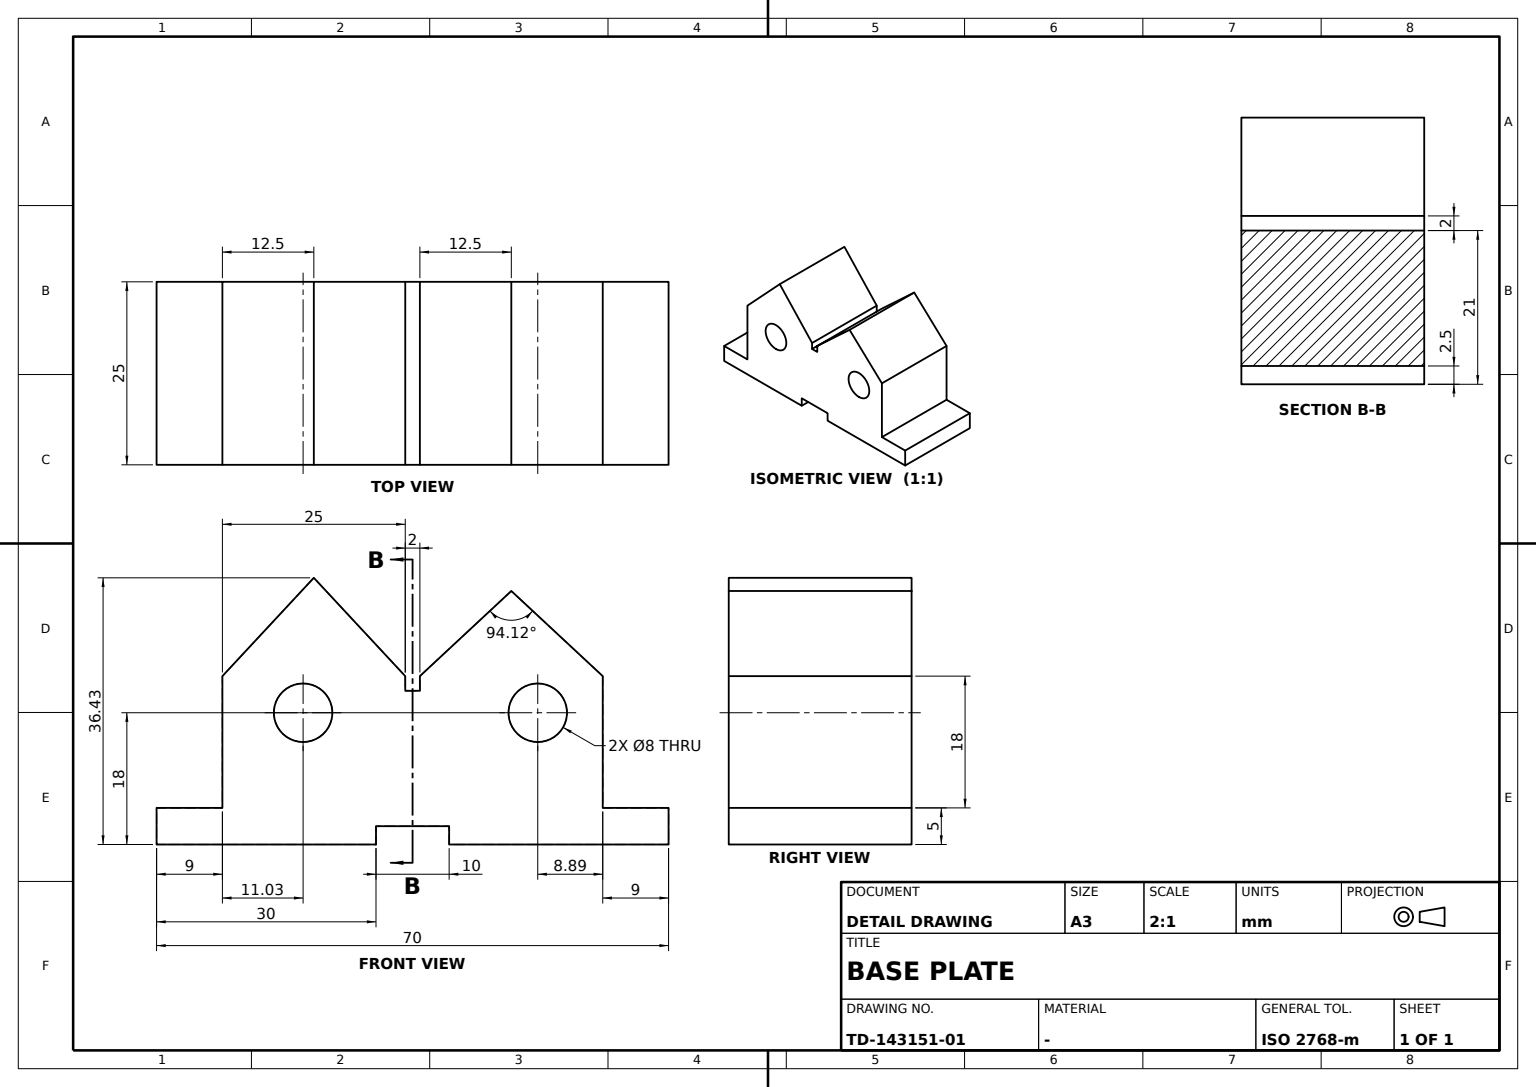
ISO-10303-21;
HEADER;
FILE_DESCRIPTION((''),'2;1');
FILE_NAME('','',(''),(''),'','','');
FILE_SCHEMA(('AUTOMOTIVE_DESIGN'));
ENDSEC;
DATA;
#1=APPLICATION_CONTEXT('');
#2=PRODUCT_CONTEXT('',#1,'mechanical');
#3=PRODUCT('','','',(#2));
#4=PRODUCT_DEFINITION_FORMATION('','',#3);
#5=PRODUCT_DEFINITION_CONTEXT('',#1,'design');
#6=PRODUCT_DEFINITION('','',#4,#5);
#7=PRODUCT_DEFINITION_SHAPE('','',#6);
#8=(LENGTH_UNIT()NAMED_UNIT(*)SI_UNIT(.MILLI.,.METRE.));
#9=(NAMED_UNIT(*)PLANE_ANGLE_UNIT()SI_UNIT($,.RADIAN.));
#10=(NAMED_UNIT(*)SI_UNIT($,.STERADIAN.)SOLID_ANGLE_UNIT());
#11=UNCERTAINTY_MEASURE_WITH_UNIT(LENGTH_MEASURE(0.005),#8,'distance_accuracy_value','');
#12=(GEOMETRIC_REPRESENTATION_CONTEXT(3)GLOBAL_UNCERTAINTY_ASSIGNED_CONTEXT((#11))GLOBAL_UNIT_ASSIGNED_CONTEXT((#8,#9,#10))REPRESENTATION_CONTEXT('',''));
#13=CARTESIAN_POINT('',(-25.,-14.966636,2.5));
#14=VERTEX_POINT('',#13);
#15=CARTESIAN_POINT('',(-25.,-14.966636,6.5));
#16=DIRECTION('',(1.,0.,0.));
#17=DIRECTION('',(0.,0.,-1.));
#18=AXIS2_PLACEMENT_3D('',#15,#16,#17);
#19=CIRCLE('',#18,4.);
#20=EDGE_CURVE('',#14,#14,#19,.T.);
#21=ORIENTED_EDGE('',*,*,#20,.F.);
#22=EDGE_LOOP('',(#21));
#23=FACE_BOUND('',#22,.T.);
#24=CARTESIAN_POINT('',(0.,-14.966636,2.5));
#25=VERTEX_POINT('',#24);
#26=CARTESIAN_POINT('',(0.,-14.966636,6.5));
#27=AXIS2_PLACEMENT_3D('',#26,#16,#17);
#28=CIRCLE('',#27,4.);
#29=EDGE_CURVE('',#25,#25,#28,.T.);
#30=ORIENTED_EDGE('',*,*,#29,.T.);
#31=EDGE_LOOP('',(#30));
#32=FACE_BOUND('',#31,.T.);
#33=CARTESIAN_POINT('',(-13.16,-14.966636,6.5));
#34=DIRECTION('',(0.,1.,0.));
#35=AXIS2_PLACEMENT_3D('',#33,#16,#34);
#36=CYLINDRICAL_SURFACE('',#35,4.);
#37=ADVANCED_FACE('',(#23,#32),#36,.F.);
#38=CARTESIAN_POINT('',(0.,35.,-11.5));
#39=VERTEX_POINT('',#38);
#40=CARTESIAN_POINT('',(0.,35.,-6.5));
#41=VERTEX_POINT('',#40);
#42=DIRECTION('',(0.,0.,1.));
#43=VECTOR('',#42,1000.);
#44=LINE('',#38,#43);
#45=EDGE_CURVE('',#39,#41,#44,.T.);
#46=ORIENTED_EDGE('',*,*,#45,.F.);
#47=CARTESIAN_POINT('',(-25.,35.,-11.5));
#48=VERTEX_POINT('',#47);
#49=DIRECTION('',(-1.,0.,0.));
#50=VECTOR('',#49,1000.);
#51=LINE('',#38,#50);
#52=EDGE_CURVE('',#39,#48,#51,.T.);
#53=ORIENTED_EDGE('',*,*,#52,.T.);
#54=CARTESIAN_POINT('',(-25.,35.,-6.5));
#55=VERTEX_POINT('',#54);
#56=LINE('',#47,#43);
#57=EDGE_CURVE('',#48,#55,#56,.T.);
#58=ORIENTED_EDGE('',*,*,#57,.T.);
#59=LINE('',#40,#50);
#60=EDGE_CURVE('',#41,#55,#59,.T.);
#61=ORIENTED_EDGE('',*,*,#60,.F.);
#62=EDGE_LOOP('',(#46,#53,#58,#61));
#63=FACE_BOUND('',#62,.T.);
#64=DIRECTION('',(0.,-1.,0.));
#65=AXIS2_PLACEMENT_3D('',#38,#64,#42);
#66=PLANE('',#65);
#67=ADVANCED_FACE('',(#63),#66,.F.);
#68=CARTESIAN_POINT('',(0.,26.,-6.5));
#69=VERTEX_POINT('',#68);
#70=VECTOR('',#64,1000.);
#71=LINE('',#40,#70);
#72=EDGE_CURVE('',#41,#69,#71,.T.);
#73=ORIENTED_EDGE('',*,*,#72,.F.);
#74=ORIENTED_EDGE('',*,*,#60,.T.);
#75=CARTESIAN_POINT('',(-25.,26.,-6.5));
#76=VERTEX_POINT('',#75);
#77=LINE('',#54,#70);
#78=EDGE_CURVE('',#55,#76,#77,.T.);
#79=ORIENTED_EDGE('',*,*,#78,.T.);
#80=LINE('',#68,#50);
#81=EDGE_CURVE('',#69,#76,#80,.T.);
#82=ORIENTED_EDGE('',*,*,#81,.F.);
#83=EDGE_LOOP('',(#73,#74,#79,#82));
#84=FACE_BOUND('',#83,.T.);
#85=AXIS2_PLACEMENT_3D('',#40,#17,#64);
#86=PLANE('',#85);
#87=ADVANCED_FACE('',(#84),#86,.F.);
#88=ORIENTED_EDGE('',*,*,#29,.F.);
#89=EDGE_LOOP('',(#88));
#90=FACE_BOUND('',#89,.T.);
#91=CARTESIAN_POINT('',(0.,-1.,11.5));
#92=VERTEX_POINT('',#91);
#93=CARTESIAN_POINT('',(0.,-1.,9.5));
#94=VERTEX_POINT('',#93);
#95=CARTESIAN_POINT('',(0.,-1.,0.));
#96=VECTOR('',#17,1000.);
#97=LINE('',#95,#96);
#98=EDGE_CURVE('',#92,#94,#97,.T.);
#99=ORIENTED_EDGE('',*,*,#98,.F.);
#100=CARTESIAN_POINT('',(0.,-13.5,24.931745));
#101=VERTEX_POINT('',#100);
#102=DIRECTION('',(0.,0.681260343,-0.732041218));
#103=VECTOR('',#102,1000.);
#104=LINE('',#100,#103);
#105=EDGE_CURVE('',#101,#92,#104,.T.);
#106=ORIENTED_EDGE('',*,*,#105,.F.);
#107=CARTESIAN_POINT('',(0.,-26.,11.5));
#108=VERTEX_POINT('',#107);
#109=DIRECTION('',(0.,0.681260343,0.732041218));
#110=VECTOR('',#109,1000.);
#111=LINE('',#107,#110);
#112=EDGE_CURVE('',#108,#101,#111,.T.);
#113=ORIENTED_EDGE('',*,*,#112,.F.);
#114=CARTESIAN_POINT('',(0.,-26.,-6.5));
#115=VERTEX_POINT('',#114);
#116=LINE('',#107,#96);
#117=EDGE_CURVE('',#108,#115,#116,.T.);
#118=ORIENTED_EDGE('',*,*,#117,.T.);
#119=CARTESIAN_POINT('',(0.,-35.,-6.5));
#120=VERTEX_POINT('',#119);
#121=EDGE_CURVE('',#115,#120,#71,.T.);
#122=ORIENTED_EDGE('',*,*,#121,.T.);
#123=CARTESIAN_POINT('',(0.,-35.,-11.5));
#124=VERTEX_POINT('',#123);
#125=LINE('',#119,#96);
#126=EDGE_CURVE('',#120,#124,#125,.T.);
#127=ORIENTED_EDGE('',*,*,#126,.T.);
#128=CARTESIAN_POINT('',(0.,-5.,-11.5));
#129=VERTEX_POINT('',#128);
#130=VECTOR('',#34,1000.);
#131=LINE('',#123,#130);
#132=EDGE_CURVE('',#124,#129,#131,.T.);
#133=ORIENTED_EDGE('',*,*,#132,.T.);
#134=CARTESIAN_POINT('',(0.,-5.,-9.));
#135=VERTEX_POINT('',#134);
#136=LINE('',#128,#43);
#137=EDGE_CURVE('',#129,#135,#136,.T.);
#138=ORIENTED_EDGE('',*,*,#137,.T.);
#139=CARTESIAN_POINT('',(0.,5.,-9.));
#140=VERTEX_POINT('',#139);
#141=LINE('',#134,#130);
#142=EDGE_CURVE('',#135,#140,#141,.T.);
#143=ORIENTED_EDGE('',*,*,#142,.T.);
#144=CARTESIAN_POINT('',(0.,5.,-11.5));
#145=VERTEX_POINT('',#144);
#146=LINE('',#144,#96);
#147=EDGE_CURVE('',#140,#145,#146,.T.);
#148=ORIENTED_EDGE('',*,*,#147,.T.);
#149=EDGE_CURVE('',#145,#39,#131,.T.);
#150=ORIENTED_EDGE('',*,*,#149,.T.);
#151=ORIENTED_EDGE('',*,*,#45,.T.);
#152=ORIENTED_EDGE('',*,*,#72,.T.);
#153=CARTESIAN_POINT('',(0.,26.,11.5));
#154=VERTEX_POINT('',#153);
#155=LINE('',#68,#43);
#156=EDGE_CURVE('',#69,#154,#155,.T.);
#157=ORIENTED_EDGE('',*,*,#156,.T.);
#158=CARTESIAN_POINT('',(0.,13.5,23.132889));
#159=VERTEX_POINT('',#158);
#160=DIRECTION('',(0.,0.732041218,-0.681260343));
#161=VECTOR('',#160,1000.);
#162=LINE('',#158,#161);
#163=EDGE_CURVE('',#159,#154,#162,.T.);
#164=ORIENTED_EDGE('',*,*,#163,.F.);
#165=CARTESIAN_POINT('',(0.,1.,11.5));
#166=VERTEX_POINT('',#165);
#167=DIRECTION('',(0.,0.732041218,0.681260343));
#168=VECTOR('',#167,1000.);
#169=LINE('',#165,#168);
#170=EDGE_CURVE('',#166,#159,#169,.T.);
#171=ORIENTED_EDGE('',*,*,#170,.F.);
#172=CARTESIAN_POINT('',(0.,1.,9.5));
#173=VERTEX_POINT('',#172);
#174=LINE('',#172,#43);
#175=EDGE_CURVE('',#173,#166,#174,.T.);
#176=ORIENTED_EDGE('',*,*,#175,.F.);
#177=LINE('',#93,#130);
#178=EDGE_CURVE('',#94,#173,#177,.T.);
#179=ORIENTED_EDGE('',*,*,#178,.F.);
#180=EDGE_LOOP('',(#99,#106,#113,#118,#122,#127,#133,#138,#143,#148,#150,#151,#152,#157,#164,#171,#176,#179));
#181=FACE_BOUND('',#180,.T.);
#182=CARTESIAN_POINT('',(0.,17.114063,2.5));
#183=VERTEX_POINT('',#182);
#184=CARTESIAN_POINT('',(0.,17.114063,6.5));
#185=AXIS2_PLACEMENT_3D('',#184,#16,#17);
#186=CIRCLE('',#185,4.);
#187=EDGE_CURVE('',#183,#183,#186,.T.);
#188=ORIENTED_EDGE('',*,*,#187,.F.);
#189=EDGE_LOOP('',(#188));
#190=FACE_BOUND('',#189,.T.);
#191=CARTESIAN_POINT('',(0.,0.,0.));
#192=AXIS2_PLACEMENT_3D('',#191,#16,#34);
#193=PLANE('',#192);
#194=ADVANCED_FACE('',(#90,#181,#190),#193,.T.);
#195=CARTESIAN_POINT('',(-25.,-35.,-11.5));
#196=VERTEX_POINT('',#195);
#197=LINE('',#123,#50);
#198=EDGE_CURVE('',#124,#196,#197,.T.);
#199=ORIENTED_EDGE('',*,*,#198,.F.);
#200=ORIENTED_EDGE('',*,*,#126,.F.);
#201=CARTESIAN_POINT('',(-25.,-35.,-6.5));
#202=VERTEX_POINT('',#201);
#203=LINE('',#119,#50);
#204=EDGE_CURVE('',#120,#202,#203,.T.);
#205=ORIENTED_EDGE('',*,*,#204,.T.);
#206=LINE('',#201,#96);
#207=EDGE_CURVE('',#202,#196,#206,.T.);
#208=ORIENTED_EDGE('',*,*,#207,.T.);
#209=EDGE_LOOP('',(#199,#200,#205,#208));
#210=FACE_BOUND('',#209,.T.);
#211=AXIS2_PLACEMENT_3D('',#119,#34,#17);
#212=PLANE('',#211);
#213=ADVANCED_FACE('',(#210),#212,.F.);
#214=CARTESIAN_POINT('',(-25.,-1.,9.5));
#215=VERTEX_POINT('',#214);
#216=CARTESIAN_POINT('',(-25.,1.,9.5));
#217=VERTEX_POINT('',#216);
#218=LINE('',#214,#130);
#219=EDGE_CURVE('',#215,#217,#218,.T.);
#220=ORIENTED_EDGE('',*,*,#219,.F.);
#221=LINE('',#93,#50);
#222=EDGE_CURVE('',#94,#215,#221,.T.);
#223=ORIENTED_EDGE('',*,*,#222,.F.);
#224=ORIENTED_EDGE('',*,*,#178,.T.);
#225=LINE('',#172,#50);
#226=EDGE_CURVE('',#173,#217,#225,.T.);
#227=ORIENTED_EDGE('',*,*,#226,.T.);
#228=EDGE_LOOP('',(#220,#223,#224,#227));
#229=FACE_BOUND('',#228,.T.);
#230=AXIS2_PLACEMENT_3D('',#93,#42,#34);
#231=PLANE('',#230);
#232=ADVANCED_FACE('',(#229),#231,.T.);
#233=ORIENTED_EDGE('',*,*,#98,.T.);
#234=ORIENTED_EDGE('',*,*,#222,.T.);
#235=CARTESIAN_POINT('',(-25.,-1.,11.5));
#236=VERTEX_POINT('',#235);
#237=CARTESIAN_POINT('',(-25.,-1.,0.));
#238=LINE('',#237,#96);
#239=EDGE_CURVE('',#236,#215,#238,.T.);
#240=ORIENTED_EDGE('',*,*,#239,.F.);
#241=LINE('',#91,#50);
#242=EDGE_CURVE('',#92,#236,#241,.T.);
#243=ORIENTED_EDGE('',*,*,#242,.F.);
#244=EDGE_LOOP('',(#233,#234,#240,#243));
#245=FACE_BOUND('',#244,.T.);
#246=AXIS2_PLACEMENT_3D('',#91,#64,#42);
#247=PLANE('',#246);
#248=ADVANCED_FACE('',(#245),#247,.F.);
#249=CARTESIAN_POINT('',(-25.,-13.5,24.931745));
#250=VERTEX_POINT('',#249);
#251=LINE('',#100,#50);
#252=EDGE_CURVE('',#101,#250,#251,.T.);
#253=ORIENTED_EDGE('',*,*,#252,.F.);
#254=ORIENTED_EDGE('',*,*,#105,.T.);
#255=ORIENTED_EDGE('',*,*,#242,.T.);
#256=LINE('',#249,#103);
#257=EDGE_CURVE('',#250,#236,#256,.T.);
#258=ORIENTED_EDGE('',*,*,#257,.F.);
#259=EDGE_LOOP('',(#253,#254,#255,#258));
#260=FACE_BOUND('',#259,.T.);
#261=AXIS2_PLACEMENT_3D('',#100,#167,#102);
#262=PLANE('',#261);
#263=ADVANCED_FACE('',(#260),#262,.T.);
#264=CARTESIAN_POINT('',(-25.,1.,11.5));
#265=VERTEX_POINT('',#264);
#266=LINE('',#165,#50);
#267=EDGE_CURVE('',#166,#265,#266,.T.);
#268=ORIENTED_EDGE('',*,*,#267,.T.);
#269=CARTESIAN_POINT('',(-25.,1.,0.));
#270=LINE('',#269,#96);
#271=EDGE_CURVE('',#265,#217,#270,.T.);
#272=ORIENTED_EDGE('',*,*,#271,.T.);
#273=ORIENTED_EDGE('',*,*,#226,.F.);
#274=ORIENTED_EDGE('',*,*,#175,.T.);
#275=EDGE_LOOP('',(#268,#272,#273,#274));
#276=FACE_BOUND('',#275,.T.);
#277=AXIS2_PLACEMENT_3D('',#172,#64,#42);
#278=PLANE('',#277);
#279=ADVANCED_FACE('',(#276),#278,.T.);
#280=CARTESIAN_POINT('',(-25.,5.,-9.));
#281=VERTEX_POINT('',#280);
#282=LINE('',#139,#50);
#283=EDGE_CURVE('',#140,#281,#282,.T.);
#284=ORIENTED_EDGE('',*,*,#283,.T.);
#285=CARTESIAN_POINT('',(-25.,5.,-11.5));
#286=VERTEX_POINT('',#285);
#287=CARTESIAN_POINT('',(-25.,5.,0.));
#288=LINE('',#287,#43);
#289=EDGE_CURVE('',#286,#281,#288,.T.);
#290=ORIENTED_EDGE('',*,*,#289,.F.);
#291=LINE('',#144,#50);
#292=EDGE_CURVE('',#145,#286,#291,.T.);
#293=ORIENTED_EDGE('',*,*,#292,.F.);
#294=ORIENTED_EDGE('',*,*,#147,.F.);
#295=EDGE_LOOP('',(#284,#290,#293,#294));
#296=FACE_BOUND('',#295,.T.);
#297=AXIS2_PLACEMENT_3D('',#144,#34,#17);
#298=PLANE('',#297);
#299=ADVANCED_FACE('',(#296),#298,.F.);
#300=CARTESIAN_POINT('',(-25.,17.114063,2.5));
#301=VERTEX_POINT('',#300);
#302=CARTESIAN_POINT('',(-25.,17.114063,6.5));
#303=AXIS2_PLACEMENT_3D('',#302,#16,#17);
#304=CIRCLE('',#303,4.);
#305=EDGE_CURVE('',#301,#301,#304,.T.);
#306=ORIENTED_EDGE('',*,*,#305,.F.);
#307=EDGE_LOOP('',(#306));
#308=FACE_BOUND('',#307,.T.);
#309=ORIENTED_EDGE('',*,*,#187,.T.);
#310=EDGE_LOOP('',(#309));
#311=FACE_BOUND('',#310,.T.);
#312=CARTESIAN_POINT('',(-13.16,17.114063,6.5));
#313=AXIS2_PLACEMENT_3D('',#312,#16,#34);
#314=CYLINDRICAL_SURFACE('',#313,4.);
#315=ADVANCED_FACE('',(#308,#311),#314,.F.);
#316=ORIENTED_EDGE('',*,*,#252,.T.);
#317=CARTESIAN_POINT('',(-25.,-26.,11.5));
#318=VERTEX_POINT('',#317);
#319=LINE('',#317,#110);
#320=EDGE_CURVE('',#318,#250,#319,.T.);
#321=ORIENTED_EDGE('',*,*,#320,.F.);
#322=LINE('',#107,#50);
#323=EDGE_CURVE('',#108,#318,#322,.T.);
#324=ORIENTED_EDGE('',*,*,#323,.F.);
#325=ORIENTED_EDGE('',*,*,#112,.T.);
#326=EDGE_LOOP('',(#316,#321,#324,#325));
#327=FACE_BOUND('',#326,.T.);
#328=DIRECTION('',(0.,-0.732041218,0.681260343));
#329=AXIS2_PLACEMENT_3D('',#107,#328,#109);
#330=PLANE('',#329);
#331=ADVANCED_FACE('',(#327),#330,.T.);
#332=ORIENTED_EDGE('',*,*,#137,.F.);
#333=CARTESIAN_POINT('',(-25.,-5.,-11.5));
#334=VERTEX_POINT('',#333);
#335=LINE('',#128,#50);
#336=EDGE_CURVE('',#129,#334,#335,.T.);
#337=ORIENTED_EDGE('',*,*,#336,.T.);
#338=CARTESIAN_POINT('',(-25.,-5.,-9.));
#339=VERTEX_POINT('',#338);
#340=LINE('',#333,#43);
#341=EDGE_CURVE('',#334,#339,#340,.T.);
#342=ORIENTED_EDGE('',*,*,#341,.T.);
#343=LINE('',#134,#50);
#344=EDGE_CURVE('',#135,#339,#343,.T.);
#345=ORIENTED_EDGE('',*,*,#344,.F.);
#346=EDGE_LOOP('',(#332,#337,#342,#345));
#347=FACE_BOUND('',#346,.T.);
#348=AXIS2_PLACEMENT_3D('',#128,#64,#42);
#349=PLANE('',#348);
#350=ADVANCED_FACE('',(#347),#349,.F.);
#351=ORIENTED_EDGE('',*,*,#20,.T.);
#352=EDGE_LOOP('',(#351));
#353=FACE_BOUND('',#352,.T.);
#354=ORIENTED_EDGE('',*,*,#289,.T.);
#355=LINE('',#338,#130);
#356=EDGE_CURVE('',#339,#281,#355,.T.);
#357=ORIENTED_EDGE('',*,*,#356,.F.);
#358=ORIENTED_EDGE('',*,*,#341,.F.);
#359=LINE('',#195,#130);
#360=EDGE_CURVE('',#196,#334,#359,.T.);
#361=ORIENTED_EDGE('',*,*,#360,.F.);
#362=ORIENTED_EDGE('',*,*,#207,.F.);
#363=CARTESIAN_POINT('',(-25.,-26.,-6.5));
#364=VERTEX_POINT('',#363);
#365=EDGE_CURVE('',#364,#202,#77,.T.);
#366=ORIENTED_EDGE('',*,*,#365,.F.);
#367=LINE('',#317,#96);
#368=EDGE_CURVE('',#318,#364,#367,.T.);
#369=ORIENTED_EDGE('',*,*,#368,.F.);
#370=ORIENTED_EDGE('',*,*,#320,.T.);
#371=ORIENTED_EDGE('',*,*,#257,.T.);
#372=ORIENTED_EDGE('',*,*,#239,.T.);
#373=ORIENTED_EDGE('',*,*,#219,.T.);
#374=ORIENTED_EDGE('',*,*,#271,.F.);
#375=CARTESIAN_POINT('',(-25.,13.5,23.132889));
#376=VERTEX_POINT('',#375);
#377=LINE('',#264,#168);
#378=EDGE_CURVE('',#265,#376,#377,.T.);
#379=ORIENTED_EDGE('',*,*,#378,.T.);
#380=CARTESIAN_POINT('',(-25.,26.,11.5));
#381=VERTEX_POINT('',#380);
#382=LINE('',#375,#161);
#383=EDGE_CURVE('',#376,#381,#382,.T.);
#384=ORIENTED_EDGE('',*,*,#383,.T.);
#385=LINE('',#75,#43);
#386=EDGE_CURVE('',#76,#381,#385,.T.);
#387=ORIENTED_EDGE('',*,*,#386,.F.);
#388=ORIENTED_EDGE('',*,*,#78,.F.);
#389=ORIENTED_EDGE('',*,*,#57,.F.);
#390=EDGE_CURVE('',#286,#48,#359,.T.);
#391=ORIENTED_EDGE('',*,*,#390,.F.);
#392=EDGE_LOOP('',(#354,#357,#358,#361,#362,#366,#369,#370,#371,#372,#373,#374,#379,#384,#387,#388,#389,#391));
#393=FACE_BOUND('',#392,.T.);
#394=ORIENTED_EDGE('',*,*,#305,.T.);
#395=EDGE_LOOP('',(#394));
#396=FACE_BOUND('',#395,.T.);
#397=CARTESIAN_POINT('',(-25.,0.,0.));
#398=AXIS2_PLACEMENT_3D('',#397,#16,#34);
#399=PLANE('',#398);
#400=ADVANCED_FACE('',(#353,#393,#396),#399,.F.);
#401=LINE('',#153,#50);
#402=EDGE_CURVE('',#154,#381,#401,.T.);
#403=ORIENTED_EDGE('',*,*,#402,.T.);
#404=ORIENTED_EDGE('',*,*,#383,.F.);
#405=LINE('',#158,#50);
#406=EDGE_CURVE('',#159,#376,#405,.T.);
#407=ORIENTED_EDGE('',*,*,#406,.F.);
#408=ORIENTED_EDGE('',*,*,#163,.T.);
#409=EDGE_LOOP('',(#403,#404,#407,#408));
#410=FACE_BOUND('',#409,.T.);
#411=AXIS2_PLACEMENT_3D('',#158,#109,#160);
#412=PLANE('',#411);
#413=ADVANCED_FACE('',(#410),#412,.T.);
#414=ORIENTED_EDGE('',*,*,#117,.F.);
#415=ORIENTED_EDGE('',*,*,#323,.T.);
#416=ORIENTED_EDGE('',*,*,#368,.T.);
#417=LINE('',#114,#50);
#418=EDGE_CURVE('',#115,#364,#417,.T.);
#419=ORIENTED_EDGE('',*,*,#418,.F.);
#420=EDGE_LOOP('',(#414,#415,#416,#419));
#421=FACE_BOUND('',#420,.T.);
#422=AXIS2_PLACEMENT_3D('',#107,#34,#17);
#423=PLANE('',#422);
#424=ADVANCED_FACE('',(#421),#423,.F.);
#425=ORIENTED_EDGE('',*,*,#204,.F.);
#426=ORIENTED_EDGE('',*,*,#121,.F.);
#427=ORIENTED_EDGE('',*,*,#418,.T.);
#428=ORIENTED_EDGE('',*,*,#365,.T.);
#429=EDGE_LOOP('',(#425,#426,#427,#428));
#430=FACE_BOUND('',#429,.T.);
#431=ADVANCED_FACE('',(#430),#86,.F.);
#432=ORIENTED_EDGE('',*,*,#406,.T.);
#433=ORIENTED_EDGE('',*,*,#378,.F.);
#434=ORIENTED_EDGE('',*,*,#267,.F.);
#435=ORIENTED_EDGE('',*,*,#170,.T.);
#436=EDGE_LOOP('',(#432,#433,#434,#435));
#437=FACE_BOUND('',#436,.T.);
#438=DIRECTION('',(0.,-0.681260343,0.732041218));
#439=AXIS2_PLACEMENT_3D('',#165,#438,#167);
#440=PLANE('',#439);
#441=ADVANCED_FACE('',(#437),#440,.T.);
#442=ORIENTED_EDGE('',*,*,#52,.F.);
#443=ORIENTED_EDGE('',*,*,#149,.F.);
#444=ORIENTED_EDGE('',*,*,#292,.T.);
#445=ORIENTED_EDGE('',*,*,#390,.T.);
#446=EDGE_LOOP('',(#442,#443,#444,#445));
#447=FACE_BOUND('',#446,.T.);
#448=AXIS2_PLACEMENT_3D('',#123,#42,#34);
#449=PLANE('',#448);
#450=ADVANCED_FACE('',(#447),#449,.F.);
#451=ORIENTED_EDGE('',*,*,#344,.T.);
#452=ORIENTED_EDGE('',*,*,#356,.T.);
#453=ORIENTED_EDGE('',*,*,#283,.F.);
#454=ORIENTED_EDGE('',*,*,#142,.F.);
#455=EDGE_LOOP('',(#451,#452,#453,#454));
#456=FACE_BOUND('',#455,.T.);
#457=AXIS2_PLACEMENT_3D('',#134,#42,#34);
#458=PLANE('',#457);
#459=ADVANCED_FACE('',(#456),#458,.F.);
#460=ORIENTED_EDGE('',*,*,#198,.T.);
#461=ORIENTED_EDGE('',*,*,#360,.T.);
#462=ORIENTED_EDGE('',*,*,#336,.F.);
#463=ORIENTED_EDGE('',*,*,#132,.F.);
#464=EDGE_LOOP('',(#460,#461,#462,#463));
#465=FACE_BOUND('',#464,.T.);
#466=ADVANCED_FACE('',(#465),#449,.F.);
#467=ORIENTED_EDGE('',*,*,#81,.T.);
#468=ORIENTED_EDGE('',*,*,#386,.T.);
#469=ORIENTED_EDGE('',*,*,#402,.F.);
#470=ORIENTED_EDGE('',*,*,#156,.F.);
#471=EDGE_LOOP('',(#467,#468,#469,#470));
#472=FACE_BOUND('',#471,.T.);
#473=AXIS2_PLACEMENT_3D('',#68,#64,#42);
#474=PLANE('',#473);
#475=ADVANCED_FACE('',(#472),#474,.F.);
#476=CLOSED_SHELL('',(#37,#67,#87,#194,#213,#232,#248,#263,#279,#299,#315,#331,#350,#400,#413,#424,#431,#441,#450,#459,#466,#475));
#477=MANIFOLD_SOLID_BREP('',#476);
#478=ADVANCED_BREP_SHAPE_REPRESENTATION('',(#477),#12);
#479=SHAPE_DEFINITION_REPRESENTATION(#7,#478);
ENDSEC;
END-ISO-10303-21;
